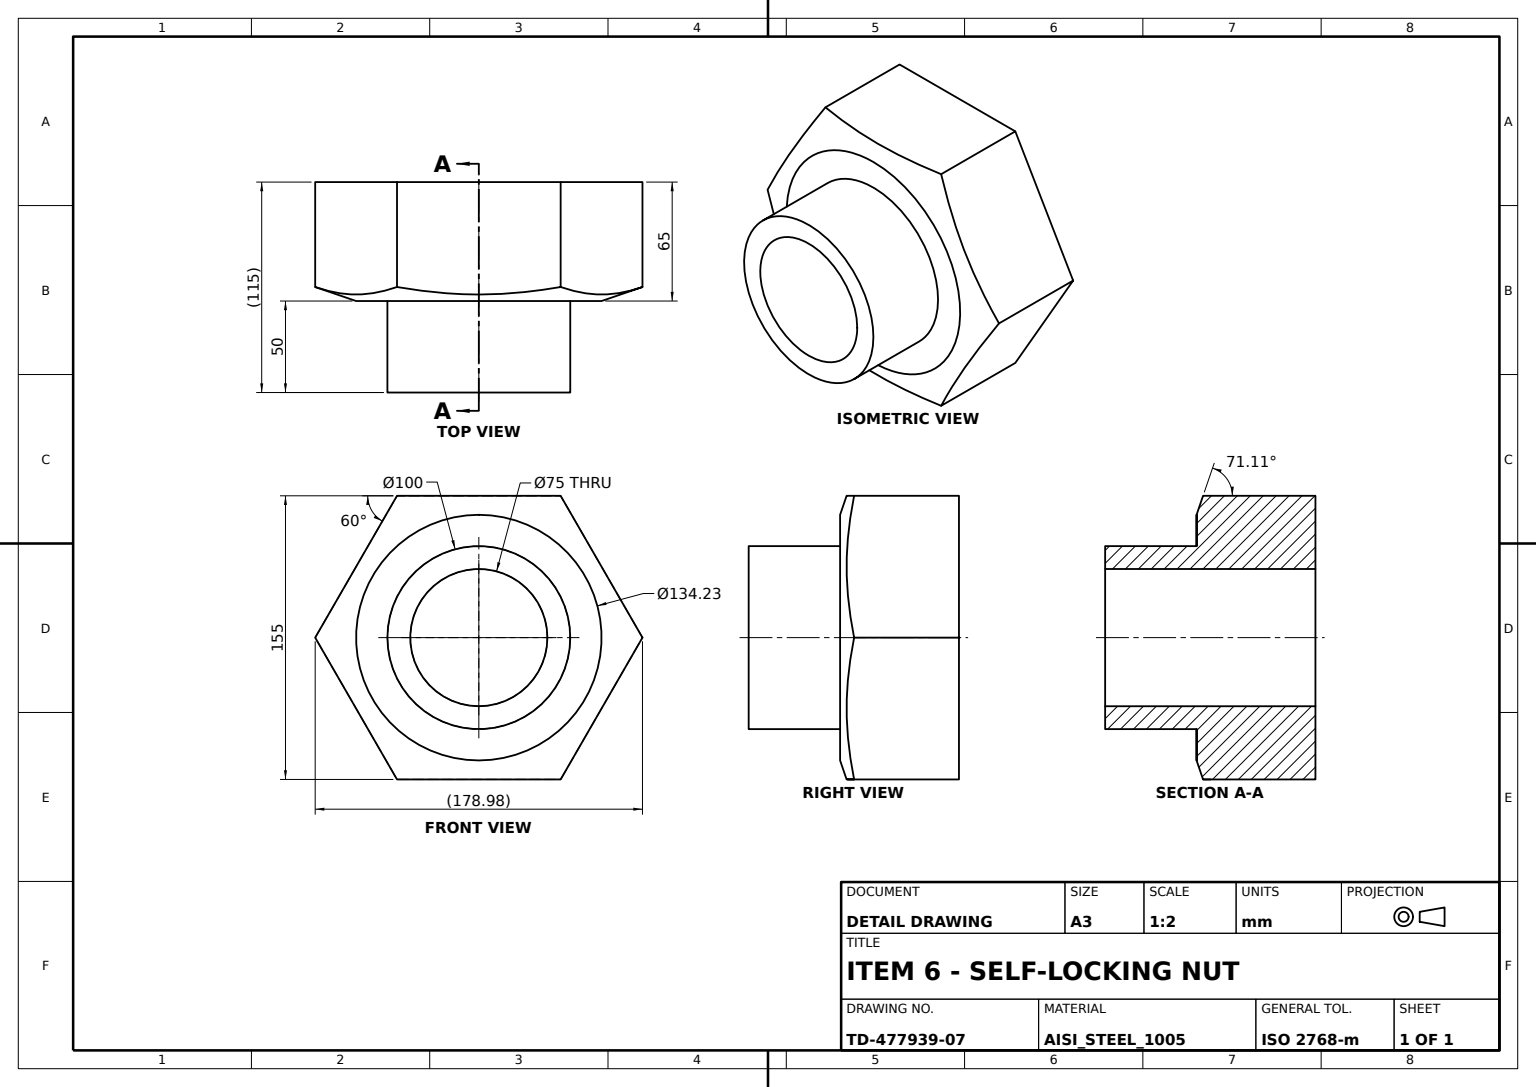
ISO-10303-21;
HEADER;
FILE_DESCRIPTION((''),'2;1');
FILE_NAME('','',(''),(''),'','','');
FILE_SCHEMA(('AUTOMOTIVE_DESIGN'));
ENDSEC;
DATA;
#1=APPLICATION_CONTEXT('');
#2=PRODUCT_CONTEXT('',#1,'mechanical');
#3=PRODUCT('','','',(#2));
#4=PRODUCT_DEFINITION_FORMATION('','',#3);
#5=PRODUCT_DEFINITION_CONTEXT('',#1,'design');
#6=PRODUCT_DEFINITION('','',#4,#5);
#7=PRODUCT_DEFINITION_SHAPE('','',#6);
#8=(LENGTH_UNIT()NAMED_UNIT(*)SI_UNIT(.MILLI.,.METRE.));
#9=(NAMED_UNIT(*)PLANE_ANGLE_UNIT()SI_UNIT($,.RADIAN.));
#10=(NAMED_UNIT(*)SI_UNIT($,.STERADIAN.)SOLID_ANGLE_UNIT());
#11=UNCERTAINTY_MEASURE_WITH_UNIT(LENGTH_MEASURE(0.005),#8,'distance_accuracy_value','');
#12=(GEOMETRIC_REPRESENTATION_CONTEXT(3)GLOBAL_UNCERTAINTY_ASSIGNED_CONTEXT((#11))GLOBAL_UNIT_ASSIGNED_CONTEXT((#8,#9,#10))REPRESENTATION_CONTEXT('',''));
#13=CARTESIAN_POINT('',(0.,-89.489292,0.));
#14=VERTEX_POINT('',#13);
#15=CARTESIAN_POINT('',(0.,-44.744646,-77.5));
#16=VERTEX_POINT('',#15);
#17=DIRECTION('',(0.,0.5,-0.866025404));
#18=VECTOR('',#17,1000.);
#19=LINE('',#13,#18);
#20=EDGE_CURVE('',#14,#16,#19,.T.);
#21=ORIENTED_EDGE('',*,*,#20,.F.);
#22=CARTESIAN_POINT('',(0.,-44.744646,77.5));
#23=VERTEX_POINT('',#22);
#24=DIRECTION('',(0.,-0.5,-0.866025404));
#25=VECTOR('',#24,1000.);
#26=LINE('',#22,#25);
#27=EDGE_CURVE('',#23,#14,#26,.T.);
#28=ORIENTED_EDGE('',*,*,#27,.F.);
#29=CARTESIAN_POINT('',(0.,44.744646,77.5));
#30=VERTEX_POINT('',#29);
#31=DIRECTION('',(0.,-1.,0.));
#32=VECTOR('',#31,1000.);
#33=LINE('',#29,#32);
#34=EDGE_CURVE('',#30,#23,#33,.T.);
#35=ORIENTED_EDGE('',*,*,#34,.F.);
#36=CARTESIAN_POINT('',(0.,89.489292,0.));
#37=VERTEX_POINT('',#36);
#38=DIRECTION('',(0.,-0.5,0.866025404));
#39=VECTOR('',#38,1000.);
#40=LINE('',#36,#39);
#41=EDGE_CURVE('',#37,#30,#40,.T.);
#42=ORIENTED_EDGE('',*,*,#41,.F.);
#43=CARTESIAN_POINT('',(0.,44.744646,-77.5));
#44=VERTEX_POINT('',#43);
#45=DIRECTION('',(0.,0.5,0.866025404));
#46=VECTOR('',#45,1000.);
#47=LINE('',#43,#46);
#48=EDGE_CURVE('',#44,#37,#47,.T.);
#49=ORIENTED_EDGE('',*,*,#48,.F.);
#50=DIRECTION('',(0.,1.,0.));
#51=VECTOR('',#50,1000.);
#52=LINE('',#15,#51);
#53=EDGE_CURVE('',#16,#44,#52,.T.);
#54=ORIENTED_EDGE('',*,*,#53,.F.);
#55=EDGE_LOOP('',(#21,#28,#35,#42,#49,#54));
#56=FACE_BOUND('',#55,.T.);
#57=CARTESIAN_POINT('',(0.,0.,-37.5));
#58=VERTEX_POINT('',#57);
#59=CARTESIAN_POINT('',(0.,0.,0.));
#60=DIRECTION('',(1.,0.,0.));
#61=DIRECTION('',(0.,0.,-1.));
#62=AXIS2_PLACEMENT_3D('',#59,#60,#61);
#63=CIRCLE('',#62,37.5);
#64=EDGE_CURVE('',#58,#58,#63,.T.);
#65=ORIENTED_EDGE('',*,*,#64,.T.);
#66=EDGE_LOOP('',(#65));
#67=FACE_BOUND('',#66,.T.);
#68=PLANE('',#62);
#69=ADVANCED_FACE('',(#56,#67),#68,.F.);
#70=CARTESIAN_POINT('',(57.345558,44.744646,77.5));
#71=VERTEX_POINT('',#70);
#72=CARTESIAN_POINT('',(57.345558,89.489292,0.));
#73=VERTEX_POINT('',#72);
#74=CARTESIAN_POINT('',(58.621298,48.473366,71.041667));
#75=CARTESIAN_POINT('',(60.695256,55.930807,58.125));
#76=CARTESIAN_POINT('',(61.823714,67.116969,38.75));
#77=CARTESIAN_POINT('',(60.695256,78.30313,19.375));
#78=CARTESIAN_POINT('',(58.621298,85.760571,6.458333));
#79=B_SPLINE_CURVE_WITH_KNOTS('',3,(#70,#74,#75,#76,#77,#78,#72),.UNSPECIFIED.,.F.,.F.,(4,1,1,1,4),(0.000000231,0.022372554,0.044744877,0.0671172,0.089489523),.UNSPECIFIED.);
#80=EDGE_CURVE('',#71,#73,#79,.T.);
#81=ORIENTED_EDGE('',*,*,#80,.T.);
#82=CARTESIAN_POINT('',(65.,89.489292,0.));
#83=DIRECTION('',(-1.,0.,0.));
#84=VECTOR('',#83,1000.);
#85=LINE('',#82,#84);
#86=EDGE_CURVE('',#73,#37,#85,.T.);
#87=ORIENTED_EDGE('',*,*,#86,.T.);
#88=ORIENTED_EDGE('',*,*,#41,.T.);
#89=CARTESIAN_POINT('',(65.,44.744646,77.5));
#90=LINE('',#89,#84);
#91=EDGE_CURVE('',#71,#30,#90,.T.);
#92=ORIENTED_EDGE('',*,*,#91,.F.);
#93=EDGE_LOOP('',(#81,#87,#88,#92));
#94=FACE_BOUND('',#93,.T.);
#95=DIRECTION('',(0.,-0.866025404,-0.5));
#96=AXIS2_PLACEMENT_3D('',#82,#95,#17);
#97=PLANE('',#96);
#98=ADVANCED_FACE('',(#94),#97,.F.);
#99=ORIENTED_EDGE('',*,*,#20,.T.);
#100=CARTESIAN_POINT('',(57.345558,-44.744646,-77.5));
#101=VERTEX_POINT('',#100);
#102=CARTESIAN_POINT('',(65.,-44.744646,-77.5));
#103=LINE('',#102,#84);
#104=EDGE_CURVE('',#101,#16,#103,.T.);
#105=ORIENTED_EDGE('',*,*,#104,.F.);
#106=CARTESIAN_POINT('',(57.345558,-89.489292,0.));
#107=VERTEX_POINT('',#106);
#108=CARTESIAN_POINT('',(58.621298,-48.473366,-71.041667));
#109=CARTESIAN_POINT('',(60.695256,-55.930807,-58.125));
#110=CARTESIAN_POINT('',(61.823714,-67.116969,-38.75));
#111=CARTESIAN_POINT('',(60.695256,-78.30313,-19.375));
#112=CARTESIAN_POINT('',(58.621298,-85.760571,-6.458333));
#113=B_SPLINE_CURVE_WITH_KNOTS('',3,(#100,#108,#109,#110,#111,#112,#106),.UNSPECIFIED.,.F.,.F.,(4,1,1,1,4),(0.000000231,0.022372554,0.044744877,0.0671172,0.089489523),.UNSPECIFIED.);
#114=EDGE_CURVE('',#101,#107,#113,.T.);
#115=ORIENTED_EDGE('',*,*,#114,.T.);
#116=CARTESIAN_POINT('',(65.,-89.489292,0.));
#117=LINE('',#116,#84);
#118=EDGE_CURVE('',#107,#14,#117,.T.);
#119=ORIENTED_EDGE('',*,*,#118,.T.);
#120=EDGE_LOOP('',(#99,#105,#115,#119));
#121=FACE_BOUND('',#120,.T.);
#122=DIRECTION('',(0.,0.866025404,0.5));
#123=AXIS2_PLACEMENT_3D('',#116,#122,#38);
#124=PLANE('',#123);
#125=ADVANCED_FACE('',(#121),#124,.F.);
#126=CARTESIAN_POINT('',(65.,0.,67.116969));
#127=VERTEX_POINT('',#126);
#128=CARTESIAN_POINT('',(65.,0.,0.));
#129=DIRECTION('',(0.,0.,1.));
#130=AXIS2_PLACEMENT_3D('',#128,#83,#129);
#131=CIRCLE('',#130,67.116969);
#132=EDGE_CURVE('',#127,#127,#131,.T.);
#133=ORIENTED_EDGE('',*,*,#132,.F.);
#134=EDGE_LOOP('',(#133));
#135=FACE_BOUND('',#134,.T.);
#136=CARTESIAN_POINT('',(65.,50.,0.));
#137=VERTEX_POINT('',#136);
#138=AXIS2_PLACEMENT_3D('',#128,#83,#50);
#139=CIRCLE('',#138,50.);
#140=EDGE_CURVE('',#137,#137,#139,.T.);
#141=ORIENTED_EDGE('',*,*,#140,.T.);
#142=EDGE_LOOP('',(#141));
#143=FACE_BOUND('',#142,.T.);
#144=AXIS2_PLACEMENT_3D('',#128,#60,#61);
#145=PLANE('',#144);
#146=ADVANCED_FACE('',(#135,#143),#145,.T.);
#147=ORIENTED_EDGE('',*,*,#132,.T.);
#148=EDGE_LOOP('',(#147));
#149=FACE_BOUND('',#148,.T.);
#150=CARTESIAN_POINT('',(57.345558,44.744646,-77.5));
#151=VERTEX_POINT('',#150);
#152=CARTESIAN_POINT('',(58.616975,-37.312477,-77.5));
#153=CARTESIAN_POINT('',(60.705154,-22.306474,-77.5));
#154=CARTESIAN_POINT('',(61.823691,0.104215,-77.5));
#155=CARTESIAN_POINT('',(60.685332,22.458415,-77.5));
#156=CARTESIAN_POINT('',(58.615622,37.320385,-77.5));
#157=B_SPLINE_CURVE_WITH_KNOTS('',3,(#100,#152,#153,#154,#155,#156,#150),.UNSPECIFIED.,.F.,.F.,(4,1,1,1,4),(0.075469683,0.098054323,0.120638963,0.143223603,0.165808243),.UNSPECIFIED.);
#158=EDGE_CURVE('',#151,#101,#157,.F.);
#159=ORIENTED_EDGE('',*,*,#158,.F.);
#160=CARTESIAN_POINT('',(58.621298,85.760571,-6.458333));
#161=CARTESIAN_POINT('',(60.695256,78.30313,-19.375));
#162=CARTESIAN_POINT('',(61.823714,67.116969,-38.75));
#163=CARTESIAN_POINT('',(60.695256,55.930807,-58.125));
#164=CARTESIAN_POINT('',(58.621298,48.473366,-71.041667));
#165=B_SPLINE_CURVE_WITH_KNOTS('',3,(#72,#160,#161,#162,#163,#164,#150),.UNSPECIFIED.,.F.,.F.,(4,1,1,1,4),(0.000000231,0.022372554,0.044744877,0.0671172,0.089489523),.UNSPECIFIED.);
#166=EDGE_CURVE('',#73,#151,#165,.T.);
#167=ORIENTED_EDGE('',*,*,#166,.F.);
#168=ORIENTED_EDGE('',*,*,#80,.F.);
#169=CARTESIAN_POINT('',(57.345558,-44.744646,77.5));
#170=VERTEX_POINT('',#169);
#171=CARTESIAN_POINT('',(58.616975,-37.312477,77.5));
#172=CARTESIAN_POINT('',(60.705154,-22.306474,77.5));
#173=CARTESIAN_POINT('',(61.823691,0.104215,77.5));
#174=CARTESIAN_POINT('',(60.685332,22.458415,77.5));
#175=CARTESIAN_POINT('',(58.615622,37.320385,77.5));
#176=B_SPLINE_CURVE_WITH_KNOTS('',3,(#169,#171,#172,#173,#174,#175,#70),.UNSPECIFIED.,.F.,.F.,(4,1,1,1,4),(0.075469683,0.098054323,0.120638963,0.143223603,0.165808243),.UNSPECIFIED.);
#177=EDGE_CURVE('',#170,#71,#176,.T.);
#178=ORIENTED_EDGE('',*,*,#177,.F.);
#179=CARTESIAN_POINT('',(58.621298,-85.760571,6.458333));
#180=CARTESIAN_POINT('',(60.695256,-78.30313,19.375));
#181=CARTESIAN_POINT('',(61.823714,-67.116969,38.75));
#182=CARTESIAN_POINT('',(60.695256,-55.930807,58.125));
#183=CARTESIAN_POINT('',(58.621298,-48.473366,71.041667));
#184=B_SPLINE_CURVE_WITH_KNOTS('',3,(#106,#179,#180,#181,#182,#183,#169),.UNSPECIFIED.,.F.,.F.,(4,1,1,1,4),(0.000000231,0.022372554,0.044744877,0.0671172,0.089489523),.UNSPECIFIED.);
#185=EDGE_CURVE('',#107,#170,#184,.T.);
#186=ORIENTED_EDGE('',*,*,#185,.F.);
#187=ORIENTED_EDGE('',*,*,#114,.F.);
#188=EDGE_LOOP('',(#159,#167,#168,#178,#186,#187));
#189=FACE_BOUND('',#188,.T.);
#190=CONICAL_SURFACE('',#130,67.116968793,1.241141809);
#191=ADVANCED_FACE('',(#149,#189),#190,.T.);
#192=ORIENTED_EDGE('',*,*,#158,.T.);
#193=ORIENTED_EDGE('',*,*,#104,.T.);
#194=ORIENTED_EDGE('',*,*,#53,.T.);
#195=CARTESIAN_POINT('',(65.,44.744646,-77.5));
#196=LINE('',#195,#84);
#197=EDGE_CURVE('',#151,#44,#196,.T.);
#198=ORIENTED_EDGE('',*,*,#197,.F.);
#199=EDGE_LOOP('',(#192,#193,#194,#198));
#200=FACE_BOUND('',#199,.T.);
#201=AXIS2_PLACEMENT_3D('',#102,#129,#31);
#202=PLANE('',#201);
#203=ADVANCED_FACE('',(#200),#202,.F.);
#204=ORIENTED_EDGE('',*,*,#64,.F.);
#205=EDGE_LOOP('',(#204));
#206=FACE_BOUND('',#205,.T.);
#207=CARTESIAN_POINT('',(115.,37.5,0.));
#208=VERTEX_POINT('',#207);
#209=CARTESIAN_POINT('',(115.,0.,0.));
#210=AXIS2_PLACEMENT_3D('',#209,#60,#50);
#211=CIRCLE('',#210,37.5);
#212=EDGE_CURVE('',#208,#208,#211,.T.);
#213=ORIENTED_EDGE('',*,*,#212,.T.);
#214=EDGE_LOOP('',(#213));
#215=FACE_BOUND('',#214,.T.);
#216=CARTESIAN_POINT('',(-35.,0.,0.));
#217=AXIS2_PLACEMENT_3D('',#216,#60,#61);
#218=CYLINDRICAL_SURFACE('',#217,37.5);
#219=ADVANCED_FACE('',(#206,#215),#218,.F.);
#220=ORIENTED_EDGE('',*,*,#140,.F.);
#221=EDGE_LOOP('',(#220));
#222=FACE_BOUND('',#221,.T.);
#223=CARTESIAN_POINT('',(115.,50.,0.));
#224=VERTEX_POINT('',#223);
#225=AXIS2_PLACEMENT_3D('',#209,#83,#50);
#226=CIRCLE('',#225,50.);
#227=EDGE_CURVE('',#224,#224,#226,.T.);
#228=ORIENTED_EDGE('',*,*,#227,.T.);
#229=EDGE_LOOP('',(#228));
#230=FACE_BOUND('',#229,.T.);
#231=AXIS2_PLACEMENT_3D('',#209,#83,#129);
#232=CYLINDRICAL_SURFACE('',#231,50.);
#233=ADVANCED_FACE('',(#222,#230),#232,.T.);
#234=ORIENTED_EDGE('',*,*,#212,.F.);
#235=EDGE_LOOP('',(#234));
#236=FACE_BOUND('',#235,.T.);
#237=ORIENTED_EDGE('',*,*,#227,.F.);
#238=EDGE_LOOP('',(#237));
#239=FACE_BOUND('',#238,.T.);
#240=PLANE('',#231);
#241=ADVANCED_FACE('',(#236,#239),#240,.F.);
#242=CARTESIAN_POINT('',(65.,-44.744646,77.5));
#243=LINE('',#242,#84);
#244=EDGE_CURVE('',#170,#23,#243,.T.);
#245=ORIENTED_EDGE('',*,*,#244,.F.);
#246=ORIENTED_EDGE('',*,*,#177,.T.);
#247=ORIENTED_EDGE('',*,*,#91,.T.);
#248=ORIENTED_EDGE('',*,*,#34,.T.);
#249=EDGE_LOOP('',(#245,#246,#247,#248));
#250=FACE_BOUND('',#249,.T.);
#251=AXIS2_PLACEMENT_3D('',#89,#61,#50);
#252=PLANE('',#251);
#253=ADVANCED_FACE('',(#250),#252,.F.);
#254=ORIENTED_EDGE('',*,*,#244,.T.);
#255=ORIENTED_EDGE('',*,*,#27,.T.);
#256=ORIENTED_EDGE('',*,*,#118,.F.);
#257=ORIENTED_EDGE('',*,*,#185,.T.);
#258=EDGE_LOOP('',(#254,#255,#256,#257));
#259=FACE_BOUND('',#258,.T.);
#260=DIRECTION('',(0.,0.866025404,-0.5));
#261=AXIS2_PLACEMENT_3D('',#242,#260,#45);
#262=PLANE('',#261);
#263=ADVANCED_FACE('',(#259),#262,.F.);
#264=ORIENTED_EDGE('',*,*,#86,.F.);
#265=ORIENTED_EDGE('',*,*,#166,.T.);
#266=ORIENTED_EDGE('',*,*,#197,.T.);
#267=ORIENTED_EDGE('',*,*,#48,.T.);
#268=EDGE_LOOP('',(#264,#265,#266,#267));
#269=FACE_BOUND('',#268,.T.);
#270=DIRECTION('',(0.,-0.866025404,0.5));
#271=AXIS2_PLACEMENT_3D('',#195,#270,#24);
#272=PLANE('',#271);
#273=ADVANCED_FACE('',(#269),#272,.F.);
#274=CLOSED_SHELL('',(#69,#98,#125,#146,#191,#203,#219,#233,#241,#253,#263,#273));
#275=MANIFOLD_SOLID_BREP('',#274);
#276=ADVANCED_BREP_SHAPE_REPRESENTATION('',(#275),#12);
#277=SHAPE_DEFINITION_REPRESENTATION(#7,#276);
ENDSEC;
END-ISO-10303-21;
